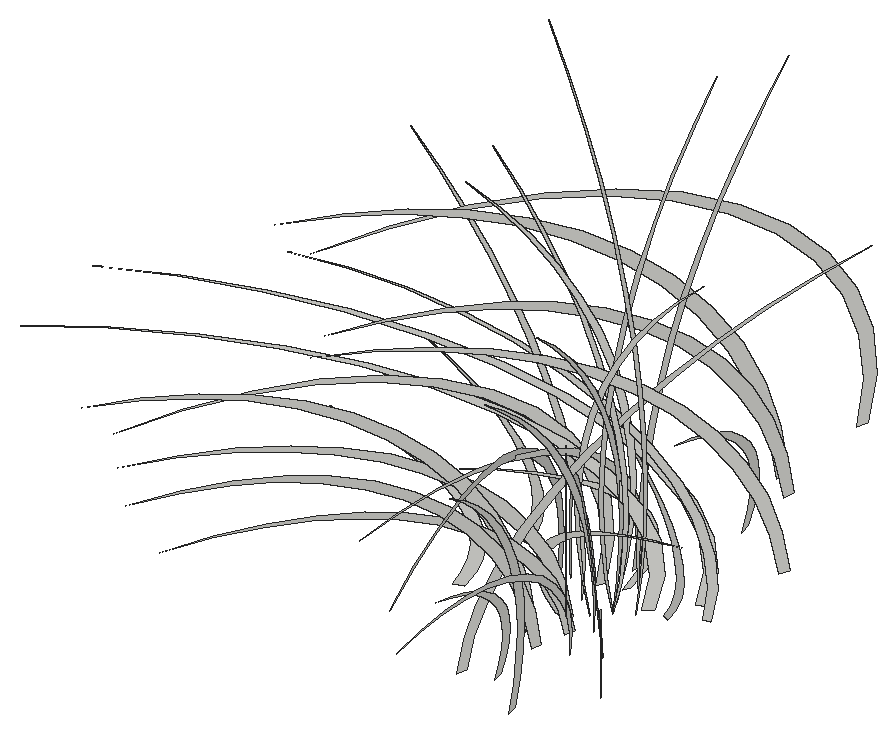
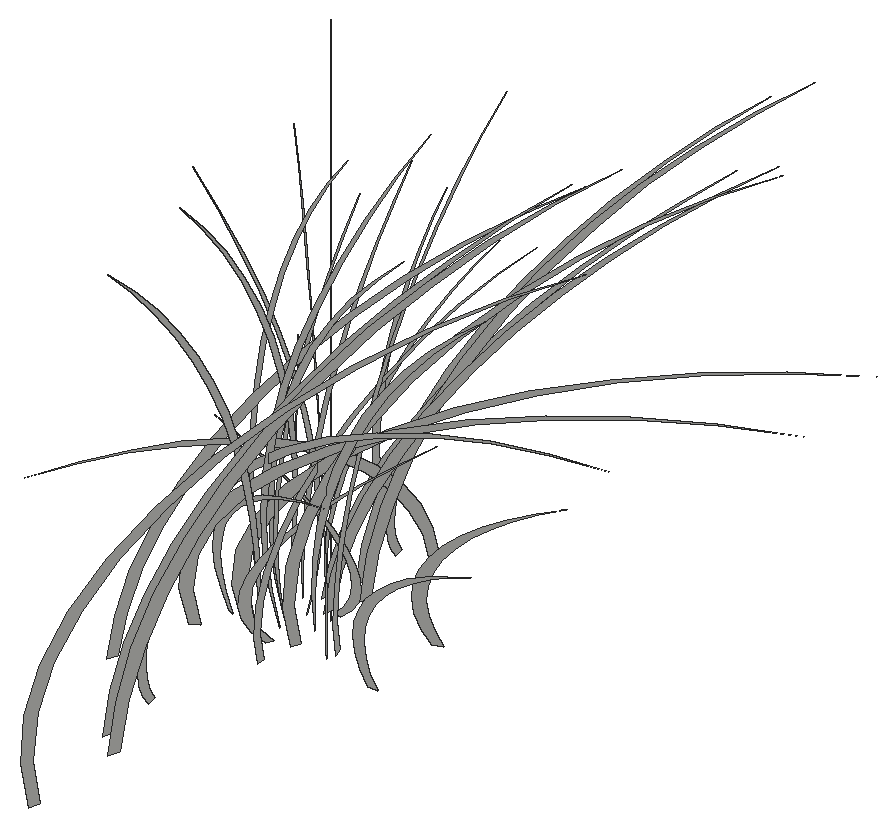
# SketchUp Ruby script. Lengths in inches.
U = 1.inch
M = Sketchup.active_model
def pt(a) = Geom::Point3d.new(a.map { |v| v * U })
def face(e, loops, mat)
  f = e.add_face(loops[0].map { |a| pt(a) })
  loops[1..].each { |l| e.add_face(l.map { |a| pt(a) }).erase! }
  f.material = f.back_material = mat if mat
  f
end
# faces: each face lists its corners as indices into pts; further lists are holes
def faces(e, pts, list, mat = nil) = list.each { |f| face(e, (f[0].is_a?(Array) ? f : [f]).map { |l| l.map { |i| pts[i] } }, mat) }
# xy, xz, yz: faces in a plane at the given z, y or x. An outline is a flat list of corners, or four numbers for a rectangle; further outlines are holes
def ring(l) = l.size == 4 ? [[l[0], l[1]], [l[2], l[1]], [l[2], l[3]], [l[0], l[3]]] : l.each_slice(2).to_a
def flat(e, list, mat, &to3) = list.each { |f| face(e, (f[0].is_a?(Array) ? f : [f]).map { |l| ring(l).map { |u, v| to3.(u, v) } }, mat) }
def xy(e, z, list, mat = nil) = flat(e, list, mat) { |x, y| [x, y, z] }
def xz(e, y, list, mat = nil) = flat(e, list, mat) { |x, z| [x, y, z] }
def yz(e, x, list, mat = nil) = flat(e, list, mat) { |y, z| [x, y, z] }
def lines(e, pts, list) = list.each { |a, b| e.add_line(pt(pts[a]), pt(pts[b])) }
# prism: a flat outline (further loops are holes) pulled along v
def prism(e, loops, v, mat = nil)
  f = face(e, loops, mat); d = Geom::Vector3d.new(v.map { |x| x * U })
  f.pushpull(f.normal.samedirection?(d) ? d.length : -d.length)
end
def box(e, o, s, mat = nil) = prism(e, [[o, [o[0] + s[0], o[1], o[2]], [o[0] + s[0], o[1] + s[1], o[2]], [o[0], o[1] + s[1], o[2]]]], [0, 0, s[2]], mat)
def at(x, y, z, deg = 0) = Geom::Transformation.translation(pt([x, y, z])) * Geom::Transformation.rotation(ORIGIN, Z_AXIS, deg.degrees)
def axes(o, x, y, z) = Geom::Transformation.new([*x, 0, *y, 0, *z, 0, *pt(o).to_a, 1])
def part(name) = M.definitions.add(name)
# library, detail: a bought-in or finely detailed component or shape, given as its bounding box
def library(name, o, s) = part(name).tap { |d| box(d.entities, o, s) }
def detail(e, o, s) = box(e.add_group.entities, o, s)
def put(e, d, t, mat = nil) = e.add_instance(d, t).tap { |i| i.material = mat if mat }
def group(e, t, mat = nil) = e.add_group.tap { |g| g.transformation = t; g.material = mat if mat }.entities
root = M.entities
g1 = group(root,at(82.85,566.125,0.02))
p = [[-0.72,-0.5,0],[-0.32,-0.22,0],[0,0,1.55],[-0.13,-0.09,3.11],[-0.71,-0.49,4.64],[-1.71,-1.2,6.1],
  [-3.13,-2.18,7.45],[-4.92,-3.43,8.67],[-7.03,-4.91,9.72],[-9.42,-6.57,10.57],[-12.03,-8.39,11.21],[-14.79,-10.32,11.62],
  [-17.63,-12.3,11.79],[-20.48,-14.29,11.71],[-17.68,-12.33,11.72],[-14.91,-10.4,11.5],[-12.23,-8.53,11.0625],[-9.7,-6.77,10.4],
  [-7.39,-5.16,9.54],[-5.34,-3.73,8.5],[-3.61,-2.52,7.3],[-2.22,-1.55,5.97],[-1.23,-0.85,4.54],[-0.63,-0.44,3.05],
  [-0.46,-0.32,1.52]]
faces(g1,p,[[0,1,2,3,4,5,6,7,8,9,10,11,12,13,14,15,16,17,18,19,20,21,22,23,24]])
g2 = group(root,at(82.85,566.125,0.02))
p = [[-0.72,-0.5,0],[-0.32,-0.22,0],[0,0,1.55],[-0.13,-0.09,3.11],[-0.71,-0.49,4.64],[-1.71,-1.2,6.1],
  [-3.13,-2.18,7.45],[-4.92,-3.43,8.67],[-7.03,-4.91,9.72],[-9.42,-6.57,10.57],[-12.03,-8.39,11.21],[-14.79,-10.32,11.62],
  [-17.63,-12.3,11.79],[-20.48,-14.29,11.71],[-17.68,-12.33,11.72],[-14.91,-10.4,11.5],[-12.23,-8.53,11.0625],[-9.7,-6.77,10.4],
  [-7.39,-5.16,9.54],[-5.34,-3.73,8.5],[-3.61,-2.52,7.3],[-2.22,-1.55,5.97],[-1.23,-0.85,4.54],[-0.63,-0.44,3.05],
  [-0.46,-0.32,1.52]]
faces(g2,p,[[0,1,2,3,4,5,6,7,8,9,10,11,12,13,14,15,16,17,18,19,20,21,22,23,24]])
g3 = group(root,at(84.35,567.57,0.02))
p = [[-0.8,-0.36,0],[-0.36,-0.16,0],[0,0,1.55],[-0.14,-0.07,3.11],[-0.78,-0.35,4.64],[-1.9,-0.86,6.1],
  [-3.48,-1.57,7.45],[-5.46,-2.47,8.67],[-7.8125,-3.53,9.72],[-10.47,-4.73,10.57],[-13.37,-6.04,11.21],[-16.43,-7.42,11.62],
  [-19.59,-8.84,11.79],[-22.76,-10.28,11.71],[-19.65,-8.87,11.72],[-16.57,-7.48,11.5],[-13.59,-6.14,11.0625],[-10.78,-4.87,10.4],
  [-8.21,-3.71,9.54],[-5.9375,-2.68,8.5],[-4.01,-1.81,7.3],[-2.47,-1.12,5.97],[-1.36,-0.61,4.54],[-0.71,-0.32,3.05],
  [-0.52,-0.23,1.52]]
faces(g3,p,[[0,1,2,3,4,5,6,7,8,9,10,11,12,13,14,15,16,17,18,19,20,21,22,23,24]])
g4 = group(root,at(76.27,566.88,0.02))
p = [[-6.32,0.62,6.98],[-5.17,0.51,6.53],[-4.12,0.4,6.05],[-3.2,0.3125,5.52],[-2.41,0.24,4.97],[-1.75,0.17,4.39],
  [-1.24,0.12,3.78],[-0.87,0.09,3.16],[-0.66,0.0625,2.53],[-0.59,0.06,1.89],[-0.68,0.07,1.25],[-0.93,0.09,0.62],
  [-1.32,0.13,0],[-0.8125,0.08,0],[-0.375,0.04,0.63],[-0.1,0.01,1.27],[0,0,1.92],[-0.07,0.01,2.57],
  [-0.31,0.03,3.21],[-0.72,0.07,3.84],[-1.29,0.125,4.45],[-2.02,0.2,5.04],[-2.9,0.28,5.59],[-3.91,0.38,6.1],
  [-5.0625,0.5,6.5625]]
faces(g4,p,[[0,1,2,3,4,5,6,7,8,9,10,11,12,13,14,15,16,17,18,19,20,21,22,23,24]])
g5 = group(root,at(76.37,563.12,0.02))
p = [[-5.95,-2.21,6.98],[-4.87,-1.81,6.53],[-3.88,-1.44,6.05],[-3.01,-1.12,5.52],[-2.27,-0.84,4.97],[-1.65,-0.61,4.39],
  [-1.16,-0.43,3.78],[-0.82,-0.3,3.16],[-0.62,-0.23,2.53],[-0.56,-0.21,1.89],[-0.65,-0.24,1.25],[-0.875,-0.33,0.62],
  [-1.25,-0.46,0],[-0.77,-0.29,0],[-0.35,-0.13,0.63],[-0.1,-0.04,1.27],[0,0,1.92],[-0.07,-0.02,2.57],
  [-0.29,-0.11,3.21],[-0.68,-0.25,3.84],[-1.21,-0.45,4.45],[-1.9,-0.71,5.04],[-2.73,-1.01,5.59],[-3.6875,-1.37,6.1],
  [-4.77,-1.77,6.5625]]
faces(g5,p,[[0,1,2,3,4,5,6,7,8,9,10,11,12,13,14,15,16,17,18,19,20,21,22,23,24]])
g6 = group(root,at(79.95,564.8,0.02))
p = [[-9.35,0.92,17.36],[-7.86,0.77,16.07],[-6.49,0.64,14.75],[-5.25,0.51,13.39],[-4.13,0.4,11.99],[-3.14,0.31,10.56],
  [-2.29,0.22,9.1],[-1.58,0.15,7.62],[-1.01,0.1,6.11],[-0.57,0.06,4.6],[-0.28,0.03,3.07],[-0.13,0.01,1.54],
  [-0.12,0.01,0],[0,0,1.54],[-0.05,0,3.09],[-0.26,0.03,4.63],[-0.64,0.0625,6.16],[-1.18,0.12,7.68],
  [-1.89,0.18,9.17],[-2.75,0.27,10.63],[-3.78,0.37,12.06],[-4.95,0.49,13.46],[-6.28,0.62,14.81],[-7.75,0.76,16.11]]
faces(g6,p,[[0,1,2,3,4,5,6,7,8,9,10,11,12,13,14,15,16,17,18,19,20,21,22,23]])
g7 = group(root,at(79.95,564.8,0.02))
p = [[-9.35,0.92,17.36],[-7.86,0.77,16.07],[-6.49,0.64,14.75],[-5.25,0.51,13.39],[-4.13,0.4,11.99],[-3.14,0.31,10.56],
  [-2.29,0.22,9.1],[-1.58,0.15,7.62],[-1.01,0.1,6.11],[-0.57,0.06,4.6],[-0.28,0.03,3.07],[-0.13,0.01,1.54],
  [-0.12,0.01,0],[0,0,1.54],[-0.05,0,3.09],[-0.26,0.03,4.63],[-0.64,0.0625,6.16],[-1.18,0.12,7.68],
  [-1.89,0.18,9.17],[-2.75,0.27,10.63],[-3.78,0.37,12.06],[-4.95,0.49,13.46],[-6.28,0.62,14.81],[-7.75,0.76,16.11]]
faces(g7,p,[[0,1,2,3,4,5,6,7,8,9,10,11,12,13,14,15,16,17,18,19,20,21,22,23]])
g8 = group(root,at(85.11,566.59,0.02))
p = [[-0.66,-0.11,0],[-0.29,-0.05,0],[0,0,1.49],[-0.12,-0.02,2.98],[-0.65,-0.11,4.45],[-1.58,-0.26,5.85],
  [-2.875,-0.47,7.15],[-4.52,-0.74,8.32],[-6.46,-1.06,9.33],[-8.66,-1.42,10.15],[-11.06,-1.81,10.76],[-13.59,-2.23,11.16],
  [-16.2,-2.65,11.32],[-18.82,-3.08,11.24],[-16.25,-2.66,11.25],[-13.7,-2.24,11.05],[-11.24,-1.84,10.62],[-8.92,-1.46,9.99],
  [-6.79,-1.11,9.16],[-4.91,-0.8,8.16],[-3.31,-0.54,7.01],[-2.04,-0.33,5.73],[-1.125,-0.18,4.36],[-0.58,-0.1,2.93],
  [-0.43,-0.07,1.46]]
faces(g8,p,[[0,1,2,3,4,5,6,7,8,9,10,11,12,13,14,15,16,17,18,19,20,21,22,23,24]])
g9 = group(root,at(79.86,582.98,0.02))
p = [[-0.28,-0.88,0],[-0.125,-0.39,0],[0,0,2.0625],[-0.05,-0.16,4.13],[-0.27,-0.86,6.16],[-0.67,-2.1,8.1],
  [-1.21,-3.83,9.91],[-1.91,-6.01,11.52],[-2.73,-8.6,12.92],[-3.66,-11.53,14.05],[-4.67,-14.72,14.9],[-5.74,-18.09,15.45],
  [-6.84,-21.56,15.67],[-7.95,-25.06,15.5625],[-6.86,-21.63,15.58],[-5.79,-18.24,15.29],[-4.75,-14.96,14.71],[-3.77,-11.87,13.83],
  [-2.87,-9.04,12.68],[-2.07,-6.54,11.3],[-1.4,-4.41,9.7],[-0.86,-2.72,7.9375],[-0.48,-1.5,6.04],[-0.25,-0.78,4.05],
  [-0.18,-0.57,2.02]]
faces(g9,p,[[0,1,2,3,4,5,6,7,8,9,10,11,12,13,14,15,16,17,18,19,20,21,22,23,24]])
g10 = group(root,at(79.91,577.5,0.02))
p = [[-6.28,-19.8,18.05],[-7.23,-22.79,18.53],[-6.3125,-19.9,17.95],[-5.43,-17.1,17.15],[-4.58,-14.4375,16.14],[-3.79,-11.93,14.93],
  [-3.05,-9.62,13.53],[-2.38,-7.52,11.96],[-1.79,-5.65,10.23],[-1.28,-4.04,8.37],[-0.86,-2.71,6.39],[-0.53,-1.68,4.32],
  [-0.3,-0.94,2.18],[-0.16,-0.52,0],[0,0,0],[-0.11,-0.35,2.23],[-0.33,-1.04,4.43],[-0.65,-2.06,6.55],
  [-1.08,-3.4,8.57],[-1.6,-5.04,10.47],[-2.21,-6.96,12.22],[-2.9,-9.13,13.8],[-3.66,-11.54,15.1875],[-4.49,-14.14,16.37],
  [-5.36,-16.91,17.33]]
faces(g10,p,[[0,1,2,3,4,5,6,7,8,9,10,11,12,13,14,15,16,17,18,19,20,21,22,23,24]])
g11 = group(root,at(79.91,577.5,0.02))
p = [[-6.28,-19.8,18.05],[-7.23,-22.79,18.53],[-6.3125,-19.9,17.95],[-5.43,-17.1,17.15],[-4.58,-14.4375,16.14],[-3.79,-11.93,14.93],
  [-3.05,-9.62,13.53],[-2.38,-7.52,11.96],[-1.79,-5.65,10.23],[-1.28,-4.04,8.37],[-0.86,-2.71,6.39],[-0.53,-1.68,4.32],
  [-0.3,-0.94,2.18],[-0.16,-0.52,0],[0,0,0],[-0.11,-0.35,2.23],[-0.33,-1.04,4.43],[-0.65,-2.06,6.55],
  [-1.08,-3.4,8.57],[-1.6,-5.04,10.47],[-2.21,-6.96,12.22],[-2.9,-9.13,13.8],[-3.66,-11.54,15.1875],[-4.49,-14.14,16.37],
  [-5.36,-16.91,17.33]]
faces(g11,p,[[0,1,2,3,4,5,6,7,8,9,10,11,12,13,14,15,16,17,18,19,20,21,22,23,24]])
g12 = group(root,at(79.84,566.75,0.02))
p = [[-0.25,-0.78,0],[-0.11,-0.35,0],[0,0,1.82],[-0.04,-0.14,3.66],[-0.24,-0.76,5.45],[-0.59,-1.86,7.17],
  [-1.07,-3.39,8.77],[-1.6875,-5.32,10.2],[-2.41,-7.61,11.43],[-3.24,-10.2,12.4375],[-4.13,-13.02,13.1875],[-5.08,-16.01,13.67],
  [-6.05,-19.08,13.87],[-7.03,-22.17,13.77],[-6.07,-19.14,13.79],[-5.12,-16.14,13.54],[-4.2,-13.24,13.01],[-3.33,-10.51,12.24],
  [-2.54,-8,11.22],[-1.83,-5.78,10],[-1.24,-3.9,8.59],[-0.76,-2.41,7.02],[-0.42,-1.33,5.34],[-0.22,-0.6875,3.59],
  [-0.16,-0.5,1.79]]
faces(g12,p,[[0,1,2,3,4,5,6,7,8,9,10,11,12,13,14,15,16,17,18,19,20,21,22,23,24]])
g13 = group(root,at(79.89,561.9,0.02))
p = [[-5.56,-17.53,15.97],[-6.4,-20.17,16.4],[-5.59,-17.61,15.89],[-4.8,-15.14,15.18],[-4.05,-12.78,14.29],[-3.35,-10.5625,13.21],
  [-2.7,-8.51,11.97],[-2.11,-6.65,10.58],[-1.59,-5,9.05],[-1.14,-3.58,7.41],[-0.76,-2.4,5.66],[-0.47,-1.48,3.82],
  [-0.26,-0.83,1.93],[-0.14,-0.46,0],[0,0,0],[-0.1,-0.31,1.98],[-0.29,-0.92,3.92],[-0.58,-1.82,5.79],
  [-0.95,-3.01,7.58],[-1.41,-4.46,9.26],[-1.95,-6.16,10.8125],[-2.5625,-8.08,12.21],[-3.24,-10.21,13.44],[-3.97,-12.51,14.49],
  [-4.75,-14.96,15.33]]
faces(g13,p,[[0,1,2,3,4,5,6,7,8,9,10,11,12,13,14,15,16,17,18,19,20,21,22,23,24]])
g14 = group(root,at(79.89,561.9,0.02))
p = [[-5.56,-17.53,15.97],[-6.4,-20.17,16.4],[-5.59,-17.61,15.89],[-4.8,-15.14,15.18],[-4.05,-12.78,14.29],[-3.35,-10.5625,13.21],
  [-2.7,-8.51,11.97],[-2.11,-6.65,10.58],[-1.59,-5,9.05],[-1.14,-3.58,7.41],[-0.76,-2.4,5.66],[-0.47,-1.48,3.82],
  [-0.26,-0.83,1.93],[-0.14,-0.46,0],[0,0,0],[-0.1,-0.31,1.98],[-0.29,-0.92,3.92],[-0.58,-1.82,5.79],
  [-0.95,-3.01,7.58],[-1.41,-4.46,9.26],[-1.95,-6.16,10.8125],[-2.5625,-8.08,12.21],[-3.24,-10.21,13.44],[-3.97,-12.51,14.49],
  [-4.75,-14.96,15.33]]
faces(g14,p,[[0,1,2,3,4,5,6,7,8,9,10,11,12,13,14,15,16,17,18,19,20,21,22,23,24]])
g15 = group(root,at(80.4,563.53,0.02))
p = [[-5.56,-17.53,12.88],[-6.4,-20.17,13.22],[-5.59,-17.61,12.8125],[-4.8,-15.14,12.24],[-4.05,-12.78,11.52],[-3.35,-10.5625,10.66],
  [-2.7,-8.51,9.66],[-2.11,-6.65,8.53],[-1.59,-5,7.3],[-1.14,-3.58,5.97],[-0.76,-2.4,4.5625],[-0.47,-1.48,3.08],
  [-0.26,-0.83,1.56],[-0.14,-0.46,0],[0,0,0],[-0.1,-0.31,1.6],[-0.29,-0.92,3.16],[-0.58,-1.82,4.67],
  [-0.95,-3.01,6.12],[-1.41,-4.46,7.47],[-1.95,-6.16,8.72],[-2.5625,-8.08,9.85],[-3.24,-10.21,10.84],[-3.97,-12.51,11.68],
  [-4.75,-14.96,12.37]]
faces(g15,p,[[0,1,2,3,4,5,6,7,8,9,10,11,12,13,14,15,16,17,18,19,20,21,22,23,24]])
g16 = group(root,at(80.4,563.53,0.02))
p = [[-5.56,-17.53,12.88],[-6.4,-20.17,13.22],[-5.59,-17.61,12.8125],[-4.8,-15.14,12.24],[-4.05,-12.78,11.52],[-3.35,-10.5625,10.66],
  [-2.7,-8.51,9.66],[-2.11,-6.65,8.53],[-1.59,-5,7.3],[-1.14,-3.58,5.97],[-0.76,-2.4,4.5625],[-0.47,-1.48,3.08],
  [-0.26,-0.83,1.56],[-0.14,-0.46,0],[0,0,0],[-0.1,-0.31,1.6],[-0.29,-0.92,3.16],[-0.58,-1.82,4.67],
  [-0.95,-3.01,6.12],[-1.41,-4.46,7.47],[-1.95,-6.16,8.72],[-2.5625,-8.08,9.85],[-3.24,-10.21,10.84],[-3.97,-12.51,11.68],
  [-4.75,-14.96,12.37]]
faces(g16,p,[[0,1,2,3,4,5,6,7,8,9,10,11,12,13,14,15,16,17,18,19,20,21,22,23,24]])
g17 = group(root,at(82.3,564.57,0.02))
p = [[-0.83,0.08,0],[-0.37,0.04,1.57],[-0.09,0.01,3.16],[0,0,4.75],[-0.09,0.01,6.34],[-0.37,0.04,7.92],
  [-0.83,0.08,9.49],[-1.47,0.14,11.04],[-2.29,0.22,12.57],[-3.29,0.32,14.05],[-4.45,0.4375,15.5],[-5.79,0.57,16.9],
  [-7.28,0.71,18.25],[-5.875,0.58,16.88],[-4.62,0.45,15.47],[-3.51,0.34,14.01],[-2.56,0.25,12.52],[-1.77,0.17,11],
  [-1.14,0.11,9.46],[-0.67,0.07,7.9],[-0.37,0.04,6.32],[-0.24,0.02,4.74],[-0.27,0.03,3.15],[-0.47,0.05,1.57]]
faces(g17,p,[[0,1,2,3,4,5,6,7,8,9,10,11,12,13,14,15,16,17,18,19,20,21,22,23]])
g18 = group(root,at(81,576.47,0.02))
p = [[-3.87,-20.41,15.34],[-4.45,-23.49,15.75],[-3.88,-20.51,15.26],[-3.34,-17.63,14.58],[-2.82,-14.88,13.72],[-2.33,-12.3,12.69],
  [-1.88,-9.91,11.5],[-1.47,-7.75,10.16],[-1.1,-5.82,8.7],[-0.79,-4.17,7.11],[-0.53,-2.8,5.43],[-0.33,-1.73,3.67],
  [-0.18,-0.97,1.86],[-0.1,-0.53,0],[0,0,0],[-0.07,-0.36,1.9],[-0.2,-1.07,3.76],[-0.4,-2.12,5.57],
  [-0.66,-3.5,7.28],[-0.98,-5.19,8.9],[-1.36,-7.17,10.39],[-1.78,-9.42,11.73],[-2.25,-11.89,12.91],[-2.76,-14.58,13.91],
  [-3.3,-17.43,14.73]]
faces(g18,p,[[0,1,2,3,4,5,6,7,8,9,10,11,12,13,14,15,16,17,18,19,20,21,22,23,24]])
g19 = group(root,at(80.85,560.99,0.02))
p = [[-3.42,-18.07,13.58],[-3.9375,-20.79,13.9375],[-3.4375,-18.15,13.5],[-2.95,-15.6,12.9],[-2.49,-13.17,12.14],[-2.0625,-10.89,11.23],
  [-1.66,-8.77,10.18],[-1.3,-6.86,8.99],[-0.98,-5.15,7.7],[-0.7,-3.6875,6.29],[-0.47,-2.48,4.81],[-0.29,-1.53,3.25],
  [-0.16,-0.86,1.64],[-0.09,-0.47,0],[0,0,0],[-0.06,-0.32,1.68],[-0.18,-0.95,3.33],[-0.36,-1.88,4.92],
  [-0.59,-3.1,6.45],[-0.87,-4.6,7.875],[-1.2,-6.35,9.19],[-1.58,-8.33,10.38],[-1.99,-10.53,11.43],[-2.44,-12.9,12.3125],
  [-2.92,-15.42,13.03]]
faces(g19,p,[[0,1,2,3,4,5,6,7,8,9,10,11,12,13,14,15,16,17,18,19,20,21,22,23,24]])
g20 = group(root,at(81.16,562.67,0.02))
p = [[-3.42,-18.07,10.95],[-3.9375,-20.79,11.24],[-3.4375,-18.15,10.89],[-2.95,-15.6,10.41],[-2.49,-13.17,9.79],[-2.0625,-10.89,9.06],
  [-1.66,-8.77,8.21],[-1.3,-6.86,7.25],[-0.98,-5.15,6.21],[-0.7,-3.6875,5.08],[-0.47,-2.48,3.875],[-0.29,-1.53,2.62],
  [-0.16,-0.86,1.32],[-0.09,-0.47,0],[0,0,0],[-0.06,-0.32,1.36],[-0.18,-0.95,2.69],[-0.36,-1.88,3.97],
  [-0.59,-3.1,5.2],[-0.87,-4.6,6.35],[-1.2,-6.35,7.41],[-1.58,-8.33,8.37],[-1.99,-10.53,9.21],[-2.44,-12.9,9.93],
  [-2.92,-15.42,10.51]]
faces(g20,p,[[0,1,2,3,4,5,6,7,8,9,10,11,12,13,14,15,16,17,18,19,20,21,22,23,24]])
g21 = group(root,at(81.22,567.73,0.02))
p = [[-3.77,-7.5,6.98],[-3.06,-6.08,6.53],[-2.41,-4.79,6.05],[-1.83,-3.65,5.52],[-1.34,-2.67,4.97],[-0.93,-1.86,4.39],
  [-0.61,-1.22,3.78],[-0.39,-0.77,3.16],[-0.25,-0.5,2.53],[-0.22,-0.43,1.89],[-0.27,-0.54,1.25],[-0.42,-0.84,0.62],
  [-0.67,-1.33,0],[-0.51,-1.01,0],[-0.23,-0.45,0.61],[-0.05,-0.1,1.24],[0.02,0.05,1.88],[-0.01,-0.02,2.53],
  [-0.14,-0.29,3.17],[-0.39,-0.77,3.8],[-0.73,-1.44,4.41],[-1.16,-2.31,4.99],[-1.69,-3.37,5.55],[-2.3125,-4.59,6.07],
  [-3.01,-5.98,6.55]]
faces(g21,p,[[0,1,2,3,4,5,6,7,8,9,10,11,12,13,14,15,16,17,18,19,20,21,22,23,24]])
g22 = group(root,at(82.99,564.88,0.02))
p = [[-0.79,0.29,0],[-0.35,0.13,2],[-0.09,0.03,4.03],[0,0,6.06],[-0.09,0.03,8.09],[-0.35,0.125,10.11],
  [-0.78,0.28,12.11],[-1.39,0.5,14.09],[-2.16,0.78,16.03],[-3.11,1.125,17.93],[-4.21,1.52,19.78],[-5.47,1.98,21.57],
  [-6.88,2.49,23.29],[-5.55,2.01,21.54],[-4.36,1.58,19.73],[-3.32,1.2,17.88],[-2.42,0.875,15.98],[-1.67,0.6,14.04],
  [-1.07,0.39,12.07],[-0.63,0.23,10.07],[-0.35,0.125,8.0625],[-0.22,0.08,6.04],[-0.25,0.09,4.02],[-0.44,0.16,2]]
faces(g22,p,[[0,1,2,3,4,5,6,7,8,9,10,11,12,13,14,15,16,17,18,19,20,21,22,23]])
g23 = group(root,at(81.38,566.19,0.02))
p = [[-0.36,-0.76,0],[-0.16,-0.34,1.74],[-0.04,-0.09,3.5],[0,0,5.27],[-0.04,-0.08,7.04],[-0.16,-0.33,8.79],
  [-0.36,-0.75,10.54],[-0.64,-1.33,12.26],[-0.99,-2.08,13.95],[-1.42,-2.98,15.6],[-1.93,-4.04,17.21],[-2.5,-5.25,18.76],
  [-3.15,-6.6,20.26],[-2.54,-5.33,18.74],[-2,-4.1875,17.17],[-1.52,-3.18,15.55],[-1.11,-2.32,13.9],[-0.76,-1.6,12.21],
  [-0.49,-1.03,10.5],[-0.29,-0.61,8.76],[-0.16,-0.34,7.02],[-0.1,-0.21,5.26],[-0.12,-0.24,3.5],[-0.2,-0.42,1.74]]
faces(g23,p,[[0,1,2,3,4,5,6,7,8,9,10,11,12,13,14,15,16,17,18,19,20,21,22,23]])
g24 = group(root,at(79.89,568.48,0.02))
p = [[0.04,-0.67,0],[0.02,-0.3,0],[0,0,1.29],[0.01,-0.12,2.6],[0.04,-0.66,3.87],[0.1,-1.59,5.09],
  [0.1875,-2.91,6.22],[0.3,-4.57,7.24],[0.42,-6.54,8.12],[0.57,-8.76,8.83],[0.72,-11.18,9.36],[0.89,-13.74,9.71],
  [1.06,-16.38,9.84],[1.23,-19.04,9.78],[1.0625,-16.43,9.79],[0.9,-13.86,9.61],[0.74,-11.37,9.24],[0.58,-9.02,8.6875],
  [0.44,-6.87,7.97],[0.32,-4.97,7.1],[0.22,-3.35,6.1],[0.13,-2.07,4.99],[0.07,-1.14,3.79],[0.04,-0.59,2.55],
  [0.03,-0.43,1.27]]
faces(g24,p,[[0,1,2,3,4,5,6,7,8,9,10,11,12,13,14,15,16,17,18,19,20,21,22,23,24]])
g25 = group(root,at(79.89,568.48,0.02))
p = [[0.04,-0.67,0],[0.02,-0.3,0],[0,0,1.29],[0.01,-0.12,2.6],[0.04,-0.66,3.87],[0.1,-1.59,5.09],
  [0.1875,-2.91,6.22],[0.3,-4.57,7.24],[0.42,-6.54,8.12],[0.57,-8.76,8.83],[0.72,-11.18,9.36],[0.89,-13.74,9.71],
  [1.06,-16.38,9.84],[1.23,-19.04,9.78],[1.0625,-16.43,9.79],[0.9,-13.86,9.61],[0.74,-11.37,9.24],[0.58,-9.02,8.6875],
  [0.44,-6.87,7.97],[0.32,-4.97,7.1],[0.22,-3.35,6.1],[0.13,-2.07,4.99],[0.07,-1.14,3.79],[0.04,-0.59,2.55],
  [0.03,-0.43,1.27]]
faces(g25,p,[[0,1,2,3,4,5,6,7,8,9,10,11,12,13,14,15,16,17,18,19,20,21,22,23,24]])
g26 = group(root,at(84.5,565.19,0.02))
p = [[-7.84,3.02,8.02],[-6.35,2.45,7.51],[-5,1.93,6.95],[-3.81,1.47,6.35],[-2.79,1.07,5.71],[-1.9375,0.75,5.04],
  [-1.28,0.49,4.35],[-0.8,0.31,3.63],[-0.53,0.2,2.9],[-0.45,0.17,2.17],[-0.5625,0.22,1.4375],[-0.88,0.34,0.71],
  [-1.39,0.54,0],[-1.05,0.41,0],[-0.47,0.18,0.7],[-0.1,0.04,1.43],[0.05,-0.02,2.16],[-0.02,0.01,2.9],
  [-0.3,0.12,3.64],[-0.8,0.31,4.36],[-1.51,0.58,5.07],[-2.42,0.93,5.74],[-3.52,1.36,6.38],[-4.8,1.85,6.98],
  [-6.24,2.41,7.53]]
faces(g26,p,[[0,1,2,3,4,5,6,7,8,9,10,11,12,13,14,15,16,17,18,19,20,21,22,23,24]])
g27 = group(root,at(84.69,571.57,0.02))
p = [[-7.01,-17,14.81],[-8.0625,-19.56,15.2],[-7.04,-17.08,14.73],[-6.05,-14.68,14.07],[-5.11,-12.39,13.24],[-4.22,-10.24,12.25],
  [-3.4,-8.26,11.1],[-2.66,-6.45,9.81],[-2,-4.85,8.39],[-1.43,-3.47,6.86],[-0.96,-2.33,5.24],[-0.59,-1.4375,3.55],
  [-0.33,-0.81,1.79],[-0.18,-0.44,0],[0,0,0],[-0.125,-0.3,1.83],[-0.37,-0.89,3.63],[-0.73,-1.77,5.37],
  [-1.2,-2.92,7.03],[-1.78,-4.32,8.59],[-2.46,-5.97,10.02],[-3.23,-7.84,11.32],[-4.08,-9.91,12.46],[-5,-12.14,13.43],
  [-5.98,-14.51,14.21]]
faces(g27,p,[[0,1,2,3,4,5,6,7,8,9,10,11,12,13,14,15,16,17,18,19,20,21,22,23,24]])
g28 = group(root,at(81.46,563.8125,0.02))
yz(g28,0,[[0.84,0,0.375,1.81,0.09,3.625,0,5.46,0.09,7.29,0.37,9.11,0.83,10.91,1.48,12.69,2.3,14.44,3.3,16.15,4.47,17.82,5.8125,19.43,7.3125,20.98,5.9,19.4,4.64,17.78,3.53,16.11,2.57,14.39,1.78,12.65,1.14,10.87,0.67,9.08,0.37,7.26,0.24,5.44,0.27,3.625,0.47,1.81]])
g29 = group(root,at(81.46,566.17,0.02))
yz(g29,0,[[0.12,0,0,1.77,0.05,3.55,0.26,5.32,0.64,7.08,1.1875,8.82,1.9,10.54,2.77,12.22,3.79,13.87,4.98,15.47,6.31,17.02,7.78,18.52,9.4,19.95,7.9,18.48,6.52,16.95,5.27,15.39,4.15,13.78,3.16,12.13,2.3,10.46,1.59,8.75,1.01,7.03,0.57,5.28,0.28,3.53,0.13,1.77]])
g30 = group(root,at(80.88,559.03,0.02))
p = [[1.29,-6.22,5.93],[1.05,-5.08,5.55],[0.84,-4.06,5.14],[0.65,-3.15,4.7],[0.49,-2.37,4.22],[0.36,-1.72,3.73],
  [0.25,-1.22,3.21],[0.18,-0.86,2.6875],[0.13,-0.65,2.15],[0.12,-0.58,1.61],[0.14,-0.67,1.0625],[0.1875,-0.91,0.53],
  [0.27,-1.3,0],[0.17,-0.8,0],[0.08,-0.37,0.53],[0.02,-0.1,1.08],[0,0,1.63],[0.01,-0.07,2.18],
  [0.0625,-0.3,2.73],[0.15,-0.71,3.27],[0.26,-1.27,3.79],[0.41,-1.99,4.28],[0.59,-2.85,4.75],[0.8,-3.85,5.18],
  [1.03,-4.98,5.58]]
faces(g30,p,[[0,1,2,3,4,5,6,7,8,9,10,11,12,13,14,15,16,17,18,19,20,21,22,23,24]])
g31 = group(root,at(79.7,557.22,0.02))
p = [[3.42,18.07,10.95],[3.9375,20.79,11.24],[3.4375,18.15,10.89],[2.95,15.6,10.41],[2.49,13.17,9.79],[2.0625,10.89,9.06],
  [1.66,8.77,8.21],[1.3,6.86,7.25],[0.98,5.15,6.21],[0.7,3.6875,5.08],[0.47,2.48,3.875],[0.29,1.53,2.62],
  [0.16,0.86,1.32],[0.09,0.47,0],[0,0,0],[0.06,0.32,1.36],[0.18,0.95,2.69],[0.36,1.88,3.97],
  [0.59,3.1,5.2],[0.87,4.6,6.35],[1.2,6.35,7.41],[1.58,8.33,8.37],[1.99,10.53,9.21],[2.44,12.9,9.93],
  [2.92,15.42,10.51]]
faces(g31,p,[[0,1,2,3,4,5,6,7,8,9,10,11,12,13,14,15,16,17,18,19,20,21,22,23,24]])
g32 = group(root,at(81.03,574.26,0.02))
p = [[1.45,-7.03,6.7],[1.1875,-5.75,6.27],[0.95,-4.58,5.81],[0.74,-3.56,5.31],[0.55,-2.68,4.77],[0.4,-1.95,4.21],
  [0.28,-1.375,3.63],[0.2,-0.97,3.03],[0.15,-0.73,2.43],[0.14,-0.66,1.8125],[0.16,-0.76,1.2],[0.21,-1.03,0.59],
  [0.3,-1.47,0],[0.1875,-0.91,0],[0.09,-0.42,0.6],[0.02,-0.11,1.22],[0,0,1.84],[0.02,-0.08,2.47],
  [0.07,-0.34,3.09],[0.16,-0.8,3.69],[0.3,-1.43,4.28],[0.46,-2.24,4.84],[0.67,-3.22,5.37],[0.9,-4.35,5.86],
  [1.16,-5.625,6.3]]
faces(g32,p,[[0,1,2,3,4,5,6,7,8,9,10,11,12,13,14,15,16,17,18,19,20,21,22,23,24]])
g33 = group(root,at(81.29,565.47,0.02))
p = [[0.17,-0.82,0],[0.08,-0.37,1.34],[0.02,-0.09,2.68],[0,0,4.03],[0.02,-0.09,5.39],[0.07,-0.36,6.73],
  [0.17,-0.81,8.07],[0.3,-1.45,9.39],[0.47,-2.25,10.68],[0.67,-3.23,11.95],[0.91,-4.38,13.18],[1.18,-5.69,14.37],
  [1.48,-7.16,15.51],[1.19,-5.78,14.35],[0.9375,-4.54,13.15],[0.71,-3.45,11.91],[0.52,-2.52,10.64],[0.36,-1.74,9.35],
  [0.23,-1.12,8.04],[0.14,-0.66,6.71],[0.08,-0.36,5.37],[0.05,-0.23,4.03],[0.05,-0.26,2.68],[0.1,-0.46,1.34]]
faces(g33,p,[[0,1,2,3,4,5,6,7,8,9,10,11,12,13,14,15,16,17,18,19,20,21,22,23]])
g34 = group(root,at(77.79,566.1875,0.02))
p = [[0.34,-0.81,0],[0.15,-0.36,0],[0,0,1.55],[0.0625,-0.15,3.11],[0.34,-0.79,4.64],[0.82,-1.92,6.1],
  [1.5,-3.51,7.45],[2.35,-5.51,8.67],[3.36,-7.89,9.72],[4.51,-10.57,10.57],[5.75,-13.49,11.21],[7.07,-16.58,11.62],
  [8.43,-19.77,11.79],[9.8,-22.97,11.71],[8.46,-19.83,11.72],[7.13,-16.72,11.5],[5.85,-13.72,11.0625],[4.64,-10.88,10.4],
  [3.54,-8.29,9.54],[2.56,-5.99,8.5],[1.73,-4.04,7.3],[1.0625,-2.49,5.97],[0.59,-1.375,4.54],[0.3,-0.71,3.05],
  [0.22,-0.52,1.52]]
faces(g34,p,[[0,1,2,3,4,5,6,7,8,9,10,11,12,13,14,15,16,17,18,19,20,21,22,23,24]])
g35 = group(root,at(78.59,563.51,0.02))
p = [[8.29,-1.375,5.93],[6.71,-1.11,5.55],[5.29,-0.88,5.14],[4.03,-0.67,4.7],[2.95,-0.49,4.22],[2.05,-0.34,3.73],
  [1.35,-0.22,3.21],[0.85,-0.14,2.6875],[0.56,-0.09,2.15],[0.47,-0.08,1.61],[0.6,-0.1,1.0625],[0.93,-0.15,0.53],
  [1.47,-0.24,0],[1.11,-0.18,0],[0.5,-0.08,0.52],[0.11,-0.02,1.06],[-0.05,0.01,1.6],[0.02,0,2.15],
  [0.32,-0.05,2.69],[0.85,-0.14,3.23],[1.59,-0.26,3.75],[2.56,-0.42,4.25],[3.72,-0.62,4.72],[5.07,-0.84,5.16],
  [6.6,-1.1,5.56]]
faces(g35,p,[[0,1,2,3,4,5,6,7,8,9,10,11,12,13,14,15,16,17,18,19,20,21,22,23,24]])
g36 = group(root,at(81.77,563.17,0.02))
p = [[1.9,-9.2,14.75],[1.6,-7.74,13.66],[1.32,-6.39,12.54],[1.07,-5.16,11.38],[0.84,-4.0625,10.1875],[0.64,-3.09,8.97],
  [0.47,-2.26,7.73],[0.32,-1.56,6.47],[0.2,-0.99,5.2],[0.12,-0.5625,3.91],[0.06,-0.27,2.61],[0.03,-0.125,1.31],
  [0.02,-0.12,0],[0,0,1.3125],[0.01,-0.04,2.625],[0.05,-0.25,3.9375],[0.13,-0.625,5.24],[0.24,-1.16,6.52],
  [0.38,-1.86,7.79],[0.56,-2.71,9.04],[0.77,-3.72,10.25],[1.01,-4.875,11.4375],[1.28,-6.18,12.59],[1.58,-7.62,13.69]]
faces(g36,p,[[0,1,2,3,4,5,6,7,8,9,10,11,12,13,14,15,16,17,18,19,20,21,22,23]])
g37 = group(root,at(82.98,557.28,0.02))
p = [[1.29,-6.22,12.05],[1.05,-5.08,11.29],[0.84,-4.06,10.45],[0.65,-3.15,9.55],[0.49,-2.37,8.59],[0.36,-1.72,7.58],
  [0.25,-1.22,6.53],[0.18,-0.86,5.46],[0.13,-0.65,4.37],[0.12,-0.58,3.26],[0.14,-0.67,2.16],[0.1875,-0.91,1.07],
  [0.27,-1.3,0],[0.17,-0.8,0],[0.08,-0.37,1.08],[0.02,-0.1,2.19],[0,0,3.32],[0.01,-0.07,4.44],
  [0.0625,-0.3,5.55],[0.15,-0.71,6.64],[0.26,-1.27,7.7],[0.41,-1.99,8.7],[0.59,-2.85,9.65],[0.8,-3.85,10.54],
  [1.03,-4.98,11.34]]
faces(g37,p,[[0,1,2,3,4,5,6,7,8,9,10,11,12,13,14,15,16,17,18,19,20,21,22,23,24]])
g38 = group(root,at(80.01,564.12,0.02))
p = [[0.83,-0.12,0],[0.37,-0.05,1.48],[0.09,-0.01,2.98],[0,0,4.48],[0.09,-0.01,5.98],[0.37,-0.05,7.48],
  [0.82,-0.12,8.96],[1.46,-0.21,10.42],[2.28,-0.33,11.86],[3.27,-0.47,13.26],[4.43,-0.64,14.625],[5.75,-0.83,15.95],
  [7.24,-1.05,17.22],[5.84,-0.84,15.93],[4.59,-0.66,14.59],[3.49,-0.5,13.22],[2.55,-0.37,11.81],[1.76,-0.25,10.38],
  [1.13,-0.16,8.92],[0.67,-0.1,7.45],[0.37,-0.05,5.96],[0.23,-0.03,4.47],[0.27,-0.04,2.97],[0.47,-0.07,1.48]]
faces(g38,p,[[0,1,2,3,4,5,6,7,8,9,10,11,12,13,14,15,16,17,18,19,20,21,22,23]])
g39 = group(root,at(82.18,561.2,0.02))
p = [[3.01,-14.56,7.44],[2.6,-12.6,7.4],[2.21,-10.67,7.22],[1.82,-8.82,6.91],[1.46,-7.07,6.48],[1.125,-5.45,5.93],
  [0.83,-4.01,5.28],[0.57,-2.76,4.54],[0.36,-1.73,3.72],[0.19,-0.9375,2.84],[0.08,-0.4,1.91],[0.03,-0.13,0.96],
  [0.03,-0.13,0],[0,0,0.98],[0.04,-0.17,1.96],[0.13,-0.64,2.92],[0.29,-1.39,3.83],[0.5,-2.41,4.67],
  [0.76,-3.68,5.43],[1.07,-5.16,6.09],[1.41,-6.83,6.64],[1.79,-8.65,7.05],[2.18,-10.57,7.33],[2.6,-12.55,7.46]]
faces(g39,p,[[0,1,2,3,4,5,6,7,8,9,10,11,12,13,14,15,16,17,18,19,20,21,22,23]])
g40 = group(root,at(77.82,566.54,0.02))
p = [[0.58,-0.66,0],[0.26,-0.29,0],[0,0,1.32],[0.1,-0.12,2.64],[0.57,-0.64,3.94],[1.39,-1.5625,5.18],
  [2.53,-2.85,6.33],[3.98,-4.48,7.37],[5.69,-6.41,8.26],[7.625,-8.59,8.99],[9.73,-10.97,9.53],[11.96,-13.49,9.875],
  [14.26,-16.08,10.02],[16.57,-18.68,9.95],[14.31,-16.125,9.96],[12.06,-13.6,9.78],[9.9,-11.15,9.4],[7.85,-8.85,8.84],
  [5.98,-6.74,8.11],[4.32,-4.87,7.22],[2.92,-3.29,6.2],[1.8,-2.03,5.07],[0.99,-1.12,3.86],[0.51,-0.58,2.59],
  [0.375,-0.42,1.29]]
faces(g40,p,[[0,1,2,3,4,5,6,7,8,9,10,11,12,13,14,15,16,17,18,19,20,21,22,23,24]])
g41 = group(root,at(84.43,560.24,0.02))
p = [[3.88,-5.03,5.93],[3.17,-4.11,5.55],[2.53,-3.28,5.14],[1.97,-2.54,4.7],[1.48,-1.91,4.22],[1.07,-1.39,3.73],
  [0.76,-0.98,3.21],[0.53,-0.69,2.6875],[0.4,-0.52,2.15],[0.36,-0.47,1.61],[0.42,-0.54,1.0625],[0.57,-0.74,0.53],
  [0.8125,-1.05,0],[0.5,-0.65,0],[0.23,-0.3,0.53],[0.0625,-0.08,1.08],[0,0,1.63],[0.04,-0.06,2.18],
  [0.19,-0.25,2.73],[0.44,-0.57,3.27],[0.79,-1.03,3.79],[1.24,-1.61,4.28],[1.78,-2.3,4.75],[2.4,-3.11,5.18],
  [3.11,-4.02,5.58]]
faces(g41,p,[[0,1,2,3,4,5,6,7,8,9,10,11,12,13,14,15,16,17,18,19,20,21,22,23,24]])
g42 = group(root,at(79.61,564.0625,0.02))
p = [[0.51,-0.64,0],[0.23,-0.28,0],[0,0,1.82],[0.09,-0.11,3.66],[0.5,-0.625,5.45],[1.22,-1.52,7.17],
  [2.22,-2.77,8.77],[3.49,-4.36,10.2],[4.99,-6.23,11.43],[6.69,-8.35,12.4375],[8.54,-10.66,13.1875],[10.5,-13.11,13.67],
  [12.52,-15.625,13.87],[14.54,-18.15,13.77],[12.56,-15.67,13.79],[10.59,-13.22,13.54],[8.69,-10.84,13.01],[6.89,-8.6,12.24],
  [5.25,-6.55,11.22],[3.79,-4.74,10],[2.5625,-3.2,8.59],[1.58,-1.97,7.02],[0.87,-1.09,5.34],[0.45,-0.5625,3.59],
  [0.33,-0.41,1.79]]
faces(g42,p,[[0,1,2,3,4,5,6,7,8,9,10,11,12,13,14,15,16,17,18,19,20,21,22,23,24]])
g43 = group(root,at(79.61,564.0625,0.02))
p = [[0.51,-0.64,0],[0.23,-0.28,0],[0,0,1.82],[0.09,-0.11,3.66],[0.5,-0.625,5.45],[1.22,-1.52,7.17],
  [2.22,-2.77,8.77],[3.49,-4.36,10.2],[4.99,-6.23,11.43],[6.69,-8.35,12.4375],[8.54,-10.66,13.1875],[10.5,-13.11,13.67],
  [12.52,-15.625,13.87],[14.54,-18.15,13.77],[12.56,-15.67,13.79],[10.59,-13.22,13.54],[8.69,-10.84,13.01],[6.89,-8.6,12.24],
  [5.25,-6.55,11.22],[3.79,-4.74,10],[2.5625,-3.2,8.59],[1.58,-1.97,7.02],[0.87,-1.09,5.34],[0.45,-0.5625,3.59],
  [0.33,-0.41,1.79]]
faces(g43,p,[[0,1,2,3,4,5,6,7,8,9,10,11,12,13,14,15,16,17,18,19,20,21,22,23,24]])
